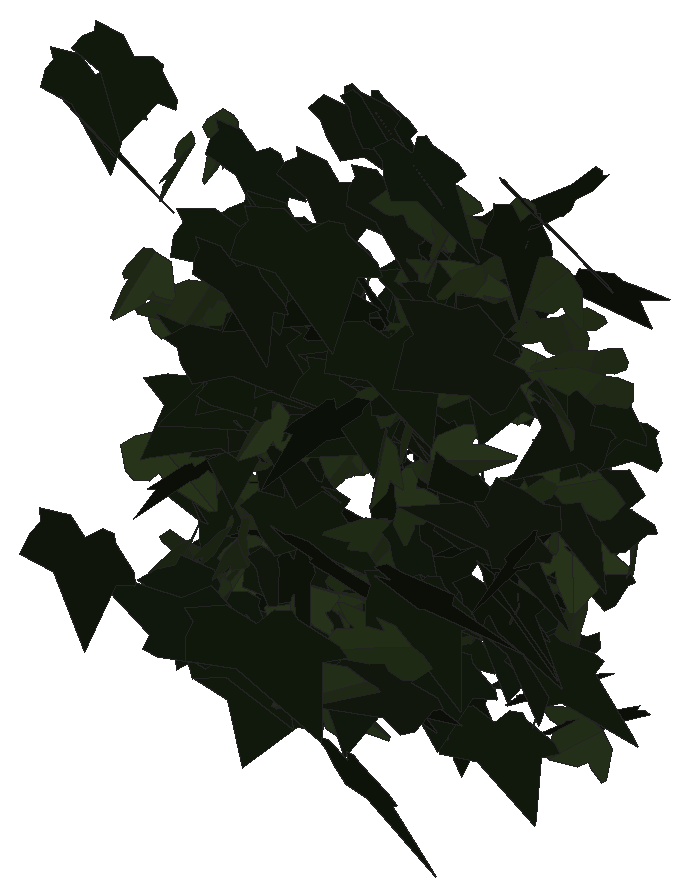
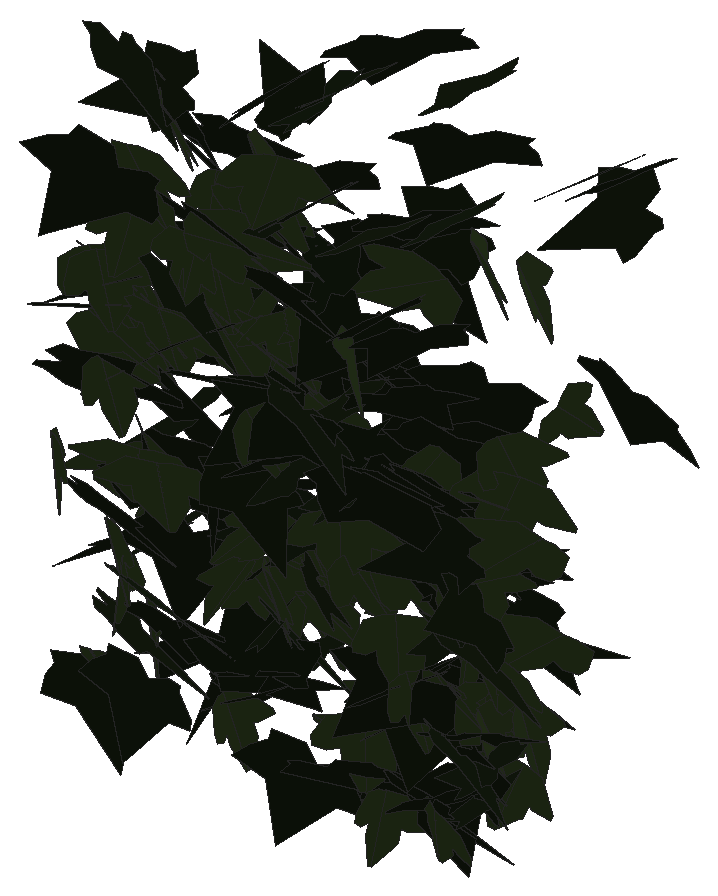
# SketchUp Ruby script. Lengths in millimetres.
U = 1.mm
M = Sketchup.active_model
def pt(a) = Geom::Point3d.new(a.map { |v| v * U })
def face(e, loops, mat)
  f = e.add_face(loops[0].map { |a| pt(a) })
  loops[1..].each { |l| e.add_face(l.map { |a| pt(a) }).erase! }
  f.material = f.back_material = mat if mat
  f
end
# faces: each face lists its corners as indices into pts; further lists are holes
def faces(e, pts, list, mat = nil) = list.each { |f| face(e, (f[0].is_a?(Array) ? f : [f]).map { |l| l.map { |i| pts[i] } }, mat) }
# xy, xz, yz: faces in a plane at the given z, y or x. An outline is a flat list of corners, or four numbers for a rectangle; further outlines are holes
def ring(l) = l.size == 4 ? [[l[0], l[1]], [l[2], l[1]], [l[2], l[3]], [l[0], l[3]]] : l.each_slice(2).to_a
def flat(e, list, mat, &to3) = list.each { |f| face(e, (f[0].is_a?(Array) ? f : [f]).map { |l| ring(l).map { |u, v| to3.(u, v) } }, mat) }
def xy(e, z, list, mat = nil) = flat(e, list, mat) { |x, y| [x, y, z] }
def xz(e, y, list, mat = nil) = flat(e, list, mat) { |x, z| [x, y, z] }
def yz(e, x, list, mat = nil) = flat(e, list, mat) { |y, z| [x, y, z] }
def lines(e, pts, list) = list.each { |a, b| e.add_line(pt(pts[a]), pt(pts[b])) }
# prism: a flat outline (further loops are holes) pulled along v
def prism(e, loops, v, mat = nil)
  f = face(e, loops, mat); d = Geom::Vector3d.new(v.map { |x| x * U })
  f.pushpull(f.normal.samedirection?(d) ? d.length : -d.length)
end
def box(e, o, s, mat = nil) = prism(e, [[o, [o[0] + s[0], o[1], o[2]], [o[0] + s[0], o[1] + s[1], o[2]], [o[0], o[1] + s[1], o[2]]]], [0, 0, s[2]], mat)
def at(x, y, z, deg = 0) = Geom::Transformation.translation(pt([x, y, z])) * Geom::Transformation.rotation(ORIGIN, Z_AXIS, deg.degrees)
def axes(o, x, y, z) = Geom::Transformation.new([*x, 0, *y, 0, *z, 0, *pt(o).to_a, 1])
def part(name) = M.definitions.add(name)
# library, detail: a bought-in or finely detailed component or shape, given as its bounding box
def library(name, o, s) = part(name).tap { |d| box(d.entities, o, s) }
def detail(e, o, s) = box(e.add_group.entities, o, s)
def put(e, d, t, mat = nil) = e.add_instance(d, t).tap { |i| i.material = mat if mat }
def group(e, t, mat = nil) = e.add_group.tap { |g| g.transformation = t; g.material = mat if mat }.entities
root = M.entities
M.materials.add("efeu1").color = [18, 25, 13]
M.materials.add("efeu2").color = [43, 57, 29]
c1 = part("ivyleaf_9")
p = [[39.1,54.8,31.7],[34.5,51.8,30.2],[-5.3,25.2,17.3],[-17.9,28.3,20.9],[-21.6,21.7,17],[-20.2,4.3,5.3],
  [-22.9,-0.3,2.5],[-17.1,-4,-0.6],[-2,-2.1,-1.2],[-0.7,-15.4,-10.1],[16.6,-22.3,-16.7],[21.1,-15.1,-12.5],
  [32.7,-10.7,-11],[46.1,-1.8,-6.6],[30.8,11.2,3.8]]
faces(c1.entities,p,[[0,1,2,3,4,5,6,7,8,9,10,11,12,13,14]],"efeu1")
c2 = part("ivyleaf_10")
p = [[0,12.8,-0.8],[-1.5,51.3,-10.9],[-4.9,51,-11.6],[-13.6,26.5,-7.3],[-13.2,15.9,-4.6],[-21.1,19.3,-7.2],
  [-29.5,16.3,-8.3],[-29.2,8.3,-6.2],[-19.7,-9.8,0.5],[-7.6,-13,4],[1,-12.2,5.8],[-0.4,51.1,-11.1],
  [-1.5,51.1,-10.9],[1,-12.4,5.9],[16.9,-12.4,3.5],[35.1,9.1,-5.1],[35,12.9,-6.1],[20.5,16.4,-4.9],
  [15.8,15,-3.8],[15.3,27.6,-7.1],[12.8,31.3,-7.8]]
faces(c2.entities,p,[[0,1,2,3,4,5,6,7,8,9,10],[11,12,0,13,14,15,16,17,18,19,20]],"efeu2")
put(root,c1,axes([5237.9,577.4,4146.6],[-0.22791,-1.24972,0.09422],[0.02085,-0.09569,-1.25528],[2.38512,-0.11858,0.01998]))
put(root,c2,axes([5260,640.4,3904.9],[0.32495,0.86733,-0.87553],[-0.70025,-0.8077,-0.87189],[-2.23853,0.37857,0.14565]))
put(root,c2,axes([5229.3,734.7,3803.5],[1.58084,0.45329,0.72541],[0.88096,0.61211,-0.91251],[-1.36903,0.91732,0.25045]))
put(root,c1,axes([5283.3,771.9,3561.8],[-0.28505,0.88899,0.74331],[-0.55358,0.69665,-0.8918],[-2.13482,-0.29935,0.13201]))
put(root,c2,axes([5256.9,721.9,3528.2],[-2.06429,0.48857,-0.04164],[0.07361,-0.01551,-1.1896],[-0.93031,-1.08533,-0.00174]))
put(root,c1,axes([5222.2,565.3,4111.4],[2.16937,-0.84957,-0.16786],[-0.25536,0.10087,-1.42163],[1.62825,1.14772,0.00069]))
put(root,c1,axes([5262.4,765.3,3729.2],[-0.69052,0.7987,-0.78771],[-0.61651,0.71802,0.87725],[2.04404,0.48638,-0.00151]))
put(root,c1,axes([5296.8,748.8,3676.6],[-0.56219,1.05041,0.51491],[-0.85878,0.38767,-1.04969],[-2.05412,-0.44956,0.29793]))
put(root,c1,axes([5254,619.8,4155.6],[-0.55085,-1.1448,0.445],[-0.10585,-0.44451,-1.1797],[2.33521,-0.29019,0.0515]))
put(root,c1,axes([5238.6,773.1,3564.9],[0.83099,-1.07671,0.08982],[0.09229,-0.07725,-1.16176],[2.05424,0.43902,0.01586]))
put(root,c2,axes([5275.1,676.9,3563.8],[0.02012,-1.23367,-0.11013],[0.02819,0.11025,-1.23362],[2.35709,0.00921,0.01569]))
put(root,c2,axes([5258.7,740.4,3658.2],[1.95897,-0.54814,0.29844],[0.5704,-0.07079,-1.16368],[1.04191,1.06935,0.07594]))
put(root,c2,axes([5245,678.7,3666.5],[1.70086,0.46056,0.67156],[1.03285,0.40653,-1.00099],[-1.15545,1.04134,0.09377]))
put(root,c1,axes([5297.6,735,3519.5],[-0.05382,-0.04278,1.25851],[-0.35098,1.24539,0.03819],[-2.37073,-0.18341,-0.03422]))
put(root,c2,axes([5274.2,701.9,3833.2],[-2.01706,-0.54132,-0.28818],[0.50917,0.10963,-1.18984],[1.05021,-1.09282,0.02338]))
put(root,c2,axes([5290.9,688.3,3864.9],[-0.85724,-1.10615,0.30759],[-0.12733,-0.30457,-1.19324],[2.18139,-0.45247,0.05123]))
put(root,c1,axes([5302.6,657.7,3674.5],[-0.53119,0.9267,-0.67379],[0.35509,-0.64747,-0.96779],[-2.1515,-0.33566,0.00662]))
put(root,c1,axes([5262,748.6,3515],[1.01788,-1.02385,-0.13399],[-0.1015,0.1233,-1.15508],[1.96258,0.53739,0.00975]))
put(root,c2,axes([5294.4,714,3568.3],[0.32806,-1.18206,0.10636],[-0.01479,-0.1086,-1.19434],[2.25875,0.17097,-0.02327]))
put(root,c2,axes([5294.2,651.9,4045.9],[0.53757,-1.20475,0.05693],[-0.00656,-0.05928,-1.23731],[2.29544,0.28197,-0.01687]))
put(root,c1,axes([5297,758,3574.9],[-1.55311,-0.84941,0.16483],[0.11329,-0.28115,-1.15413],[1.64285,-0.78362,0.23541]))
put(root,c2,axes([5304.1,727.2,3737],[-1.14837,-1.02735,0.23072],[0.10429,-0.29619,-1.17559],[2.00123,-0.57409,0.19365]))
put(root,c1,axes([5312.2,686,3734.8],[-1.35491,-0.79199,0.51244],[-0.71641,-0.35015,-1.06412],[1.64618,-0.80424,-0.04133]))
put(root,c1,axes([5308.1,709.1,3720],[-0.72384,-1.20414,-0.13162],[0.05169,0.12944,-1.26271],[2.30479,-0.38108,-0.01302]))
put(root,c1,axes([5313.1,775.2,3507],[-0.76161,-1.08531,0.1492],[-0.01712,-0.15558,-1.15586],[2.08492,-0.39774,0.04501]))
put(root,c2,axes([5306.3,775.9,3483.8],[1.58972,-0.71026,0.39583],[0.67689,-0.19116,-1.09353],[1.39162,0.90435,0.07972]))
put(root,c2,axes([5294.8,751.8,3594.9],[-0.20029,-0.10752,-1.16255],[1.26411,-0.96548,0.02917],[-1.82739,-0.65609,0.14759]))
put(root,c2,axes([5333.9,662.1,3545.3],[-0.46592,-1.18275,-0.22608],[0.02743,0.22781,-1.20741],[2.2916,-0.2432,-0.03152]))
put(root,c2,axes([5329.3,679.8,4070.3],[1.17842,-1.08302,0.07791],[0.05266,-0.07392,-1.24746],[2.06586,0.61967,-0.01264]))
put(root,c1,axes([5297.9,751.5,3775.4],[1.91409,-0.61192,0.16135],[0.28467,-0.06454,-1.17704],[1.17028,1.01654,0.0224]))
put(root,c1,axes([5362.8,700.6,3760.9],[-2.13188,-0.20027,0.3169],[-0.47549,-0.34563,-1.10155],[0.53192,-1.11163,0.2854]))
put(root,c1,axes([5351.3,736.2,3500],[1.07349,0.74499,-0.75413],[-0.92255,-0.57843,-0.93398],[-1.79421,0.74315,0.02904]))
put(root,c1,axes([5309.7,746.8,3684.9],[1.36334,-0.94,-0.05223],[-0.01949,0.05784,-1.18153],[1.79165,0.71591,0.02689]))
put(root,c1,axes([5359.2,713.3,3802.1],[-2.01308,-0.53843,0.06073],[-0.08795,-0.04308,-1.18676],[1.02748,-1.0586,0.01741]))
put(root,c2,axes([5350,762.8,3610.4],[-0.61426,-1.13811,0.01923],[0.01503,-0.02223,-1.18291],[2.16631,-0.32256,0.01366]))
put(root,c1,axes([5381.2,750.1,3484.8],[-1.9941,0.3785,0.34047],[-0.62301,0.09577,-1.11385],[-0.74206,-1.09752,0.02022]))
put(root,c2,axes([5367.8,651.2,3523],[-1.86562,0.27387,0.58187],[-1.05635,0.17549,-1.01765],[-0.61821,-1.12635,-0.01707]))
put(root,c2,axes([5350.5,704.1,3569.3],[0.84989,0.84491,-0.76393],[-0.67227,-0.67737,-0.95566],[-2.06099,0.56937,-0.0033]))
put(root,c1,axes([5368.1,703.7,3750.5],[-2.20645,-0.2236,-0.0257],[0.04676,0.00828,-1.1807],[0.4258,-1.15959,-0.00348]))
put(root,c1,axes([5357.6,633.8,3556.1],[-2.10836,-0.30583,-0.39696],[0.72036,0.12054,-1.14914],[0.62501,-1.17058,-0.01463]))
put(root,c1,axes([5354.9,738.5,3579.9],[1.2446,0.96259,-0.06883],[-0.31878,0.03132,-1.15323],[-1.80881,0.65682,0.15588]))
put(root,c1,axes([5389.9,731.6,3824.5],[-2.25643,0.12473,0.03765],[-0.08238,-0.05197,-1.19082],[-0.23389,-1.18506,0.05619]))
put(root,c1,axes([5408,547.4,3556.7],[-0.49827,0.40964,1.0866],[-2.04939,0.33134,-0.38436],[-0.82735,-1.06746,0.29768]))
put(root,c2,axes([5365.3,650.7,3611.4],[0.00245,-0.96061,-0.67602],[0.22173,0.67279,-0.9558],[2.22454,-0.066,0.09601]))
put(root,c2,axes([5389.3,720.3,3709.7],[-1.23799,-0.7406,0.69449],[-0.87674,-0.51972,-0.9857],[1.72194,-0.79707,-0.00257]))
put(root,c1,axes([5409.6,646.5,3801.2],[-0.02836,0.32803,1.17932],[-2.20002,0.38422,-0.12148],[-0.7664,-1.11507,0.30508]))
put(root,c2,axes([5376.1,756.2,3664.7],[-1.43593,-0.92194,-0.00246],[0.18958,-0.07835,-1.18455],[1.74437,-0.7504,0.12671]))
put(root,c2,axes([5374.1,613.7,3563.7],[0.76655,-1.1928,0.12568],[0.07356,-0.1196,-1.25897],[2.28152,0.40461,-0.00163]))
put(root,c2,axes([5372.8,778.4,3477.4],[-0.63948,-0.99066,-0.48377],[0.35537,0.4473,-1.04566],[2.0679,-0.38322,0.03009]))
put(root,c1,axes([5351,756,3616.3],[2.21156,0.28427,-0.00735],[-0.01443,0.00005,-1.19628],[-0.54101,1.16204,0.00185]))
put(root,c1,axes([5372.8,725.7,3704.2],[-1.82188,0.09461,-0.72432],[1.37764,-0.03746,-0.96155],[-0.18667,-1.19983,-0.0271]))
put(root,c1,axes([5365.5,761.6,3607.2],[0.38947,-1.08175,-0.44392],[0.04961,0.45477,-1.09618],[2.22484,0.17923,0.10215]))
put(root,c2,axes([5396,674.5,3763.6],[0.22483,0.57585,-1.08771],[-0.51037,-1.05441,-0.58734],[-2.28606,0.29204,0.02415]))
put(root,c2,axes([5383.9,686.5,3818.8],[-0.44911,-0.78626,-0.90793],[0.88728,0.79277,-0.80771],[2.10662,-0.50153,0.14663]))
put(root,c1,axes([5426.4,742.1,3814.4],[0.18199,0.71603,-0.96847],[-1.04944,-0.8377,-0.67379],[-2.03792,0.49532,0.26048]))
put(root,c1,axes([5379,722.6,3552.7],[-0.00877,-1.26429,-0.03826],[0.00435,0.03825,-1.2643],[2.40729,-0.00467,0.00215]))
put(root,c1,axes([5379.6,614.9,3878.1],[-0.15167,-0.47823,-1.25039],[0.56377,1.21525,-0.48368],[2.4847,-0.30493,0.03342]))
put(root,c1,axes([5388.8,654.9,4075.5],[-0.10535,-1.23831,0.35809],[0.085,-0.36005,-1.23817],[2.45184,-0.04072,0.05831]))
put(root,c1,axes([5396.5,360.9,3751.1],[-1.84525,-0.06355,-1.07431],[2.04789,-0.03196,-0.96921],[0.03582,-1.44677,0.0686]))
put(root,c1,axes([5392,709.1,3703.5],[-0.61097,-0.91042,0.83619],[0.49317,-0.89429,-0.8742],[2.30038,-0.05008,0.4095]))
put(root,c2,axes([5419.9,753.6,3534.7],[-1.89089,-0.60302,0.01928],[-0.0396,-0.00288,-1.16219],[1.14758,-0.99371,-0.00834]))
put(root,c1,axes([5443.1,729.2,3800.5],[-2.29494,-0.1099,0.15137],[-0.28902,-0.00146,-1.21077],[0.20789,-1.2153,-0.01223]))
put(root,c1,axes([5396,693.4,3581.1],[0.7215,-1.02551,-0.53719],[-0.12805,0.54478,-1.08749],[2.19959,0.3681,0.1129]))
put(root,c1,axes([5408.6,585.4,3544.7],[0.09476,-0.9833,-0.74105],[0.07131,0.74252,-0.98273],[2.34226,0.01718,0.0599]))
put(root,c2,axes([5440.4,738.2,3703.4],[-0.8309,-1.01558,0.47968],[-0.1626,-0.48313,-1.10063],[2.13141,-0.43276,0.10303]))
put(root,c1,axes([5413.7,681.5,3954],[-0.23004,-1.09468,-0.56798],[0.13159,0.56379,-1.10132],[2.34345,-0.13911,0.00609]))
put(root,c1,axes([5441.9,686.1,3876],[-1.59733,-0.89633,0.20818],[-0.30492,-0.13512,-1.22769],[1.72455,-0.8541,-0.02425]))
put(root,c1,axes([5442.9,777.7,3496.4],[-1.63597,-0.77741,-0.01579],[0.03221,0.00483,-1.15896],[1.47952,-0.85972,0.00777]))
put(root,c2,axes([5419.6,687.2,3541.6],[1.21661,0.72765,0.69517],[0.44629,0.69319,-0.9412],[-1.86255,0.64139,0.22856]))
put(root,c2,axes([5438.9,618.6,3512.1],[0.49921,-1.00435,0.55414],[0.47723,-0.50449,-1.03306],[2.13032,0.34837,0.10157]))
put(root,c1,axes([5452.7,601.3,3495.1],[-1.26317,-1.0191,0.02927],[-0.03828,-0.02184,-1.21617],[1.93998,-0.66399,-0.00493]))
put(root,c2,axes([5457.8,744.8,3748.8],[-1.78084,-0.76233,0.03479],[0.2411,-0.20945,-1.18237],[1.43223,-0.91263,0.24229]))
put(root,c1,axes([5423.6,663.8,3674.7],[0.69608,-0.87243,-0.82538],[0.40114,0.89604,-0.85372],[2.25026,0.11014,0.40751]))
put(root,c1,axes([5440,702.4,3974.9],[0.27596,-1.21425,-0.24147],[-0.05558,0.2397,-1.22288],[2.35556,0.14791,-0.00057]))
put(root,c1,axes([5441,740.4,3792.7],[0.84382,-1.13121,0.01637],[0.00249,-0.01707,-1.21499],[2.15315,0.44334,-0.00501]))
put(root,c1,axes([5435.8,577.7,4019.5],[2.39168,-0.52278,-0.12136],[-0.21303,0.0469,-1.36107],[0.99896,1.26164,0.00031]))
put(root,c2,axes([5493.6,684.7,3909.1],[-0.09238,0.68487,0.99138],[-1.41521,0.76369,-0.56398],[-1.80447,-0.63401,0.39157]))
put(root,c1,axes([5471.6,615.7,4035.2],[-1.36968,-1.05973,-0.05846],[0.0738,0.04433,-1.28098],[2.0186,-0.72068,0.00717]))
put(root,c1,axes([5463.9,695.3,4047.6],[-0.54818,-1.14377,0.45283],[0.11547,-0.47772,-1.16804],[2.33836,-0.24454,0.16383]))
put(root,c2,axes([5450.4,620.7,3974.5],[-1.66533,0.28806,-0.84956],[1.54659,-0.24813,-0.92111],[-0.72312,-1.19408,-0.01354]))
put(root,c1,axes([5496.6,716.9,3778.1],[-1.55553,-0.66662,0.5649],[-0.61723,-0.48682,-1.04371],[1.54418,-0.8661,0.15187]))
put(root,c1,axes([5479.4,759.5,3476.6],[1.28471,0.94644,0.089],[0.08238,0.07844,-1.16246],[-1.80734,0.67634,0.01028]))
put(root,c1,axes([5511.9,591.3,3988.4],[0.75224,0.52275,-1.20226],[-1.26302,-1.00316,-0.65436],[-2.15178,0.77157,-0.03622]))
put(root,c1,axes([5517.6,724.2,3848.1],[-0.18634,1.03475,0.63578],[-0.46193,0.6083,-1.02741],[-2.26474,-0.20921,0.15725]))
put(root,c1,axes([5468.9,617.5,3637.4],[-0.4806,-0.17771,-1.14255],[2.07869,-0.42056,-0.17598],[-0.7224,-1.09193,0.25373]))
put(root,c1,axes([5480.3,514.2,4079.6],[-0.90272,-0.99512,-0.72011],[0.60351,0.64657,-1.10236],[2.25854,-0.57051,0.00674]))
put(root,c2,axes([5455,674.4,3458.3],[-0.03992,-0.11471,1.23716],[2.31706,-0.24892,-0.00244],[0.47208,1.21204,0.11659]))
put(root,c2,axes([5492.1,605.5,3596.8],[-0.11916,1.13127,0.37431],[-0.01184,0.37451,-1.13292],[-2.2678,-0.0614,-0.01375]))
put(root,c2,axes([5519,714.6,3634.9],[-1.13193,-0.77398,0.67122],[-0.34215,-0.68524,-0.94944],[1.91955,-0.57854,0.22658]))
put(root,c1,axes([5509.8,730.9,3676.5],[-1.33174,0.44726,-0.83712],[1.2696,-0.50805,-0.82905],[-1.28491,-0.96555,0.04846]))
put(root,c2,axes([5523.3,694.2,3663.9],[-0.97706,-1.07875,0.23056],[-0.13089,-0.22251,-1.19423],[2.09537,-0.51692,0.03291]))
put(root,c1,axes([5491.2,675.7,3847.5],[1.25146,-1.008,-0.38591],[-0.10607,0.41957,-1.1909],[2.05148,0.63661,0.17384]))
put(root,c1,axes([5551.4,726.3,3611.6],[-1.60967,0.82767,-0.03501],[0.03983,-0.02868,-1.18336],[-1.57613,-0.84601,0.00586]))
put(root,c1,axes([5537.2,773.7,3563.1],[-1.72545,-0.72803,0.12405],[-0.08938,-0.13918,-1.16008],[1.40272,-0.90441,0.07867]))
put(root,c1,axes([5517.8,643,3922.4],[1.54915,0.88754,0.23094],[0.27093,0.18276,-1.20414],[-1.72426,0.82612,0.01828]))
put(root,c1,axes([5543,588.4,3855.2],[-0.59743,0.82169,-1.14209],[0.80672,-1.06057,-0.87954],[-2.55331,-0.52735,-0.01066]))
put(root,c2,axes([5536.5,751.7,3659.3],[1.06882,-1.05252,-0.11899],[0.01195,0.13799,-1.1909],[2.01587,0.55723,0.07015]))
put(root,c1,axes([5508.1,737.4,3725.4],[1.53365,-0.90449,0.13717],[0.30048,-0.04255,-1.20811],[1.71498,0.81631,0.08901]))
put(root,c1,axes([5533.2,644.9,3860.2],[-0.86568,-1.05863,-0.34168],[0.33066,0.297,-1.15149],[2.09114,-0.48521,0.04063]))
put(root,c2,axes([5569.5,740.8,3652.1],[-1.49094,-0.75221,0.50739],[-0.67515,-0.36306,-1.08596],[1.5894,-0.85984,0.01466]))
put(root,c1,axes([5516.4,742.1,3782.7],[0.82108,-1.11758,0.19461],[0.38181,-0.12976,-1.18991],[2.12495,0.45515,0.13861]))
put(root,c1,axes([5528.4,721.7,3841.7],[2.22595,0.32562,0.09535],[0.13299,0.10374,-1.21136],[-0.63191,1.16887,0.08095]))
put(root,c1,axes([5523.2,640.4,4181.8],[1.01346,-1.0837,-0.55234],[0.00125,0.60321,-1.18287],[2.31494,0.47411,0.24245]))
put(root,c1,axes([5535.4,695.4,4063.3],[0.03492,-1.25886,0.08215],[-0.07644,-0.0827,-1.25832],[2.39974,0.01569,-0.04128]))
put(root,c1,axes([5534.7,743.1,3622.4],[1.31326,-0.8234,-0.47872],[-0.61211,0.35499,-1.07417],[1.70623,0.76111,-0.0169]))
put(root,c1,axes([5526.8,773.6,3575.1],[2.36028,-0.40697,-0.16293],[0.29799,-0.04543,1.30522],[-0.77928,-1.25,0.00561]))
put(root,c1,axes([5529.6,678.3,3552.1],[0.61074,-1.15031,0.18653],[0.09004,-0.18045,-1.19422],[2.21603,0.32436,-0.00289]))
put(root,c1,axes([5532.7,443.5,4082.3],[0.08081,-1.24525,0.32852],[0.18294,-0.32472,-1.24326],[2.44421,0.06548,0.08219]))
put(root,c1,axes([5572.3,748.8,3766.8],[0.01859,1.16074,-0.31388],[-0.01554,-0.31382,-1.16077],[-2.28842,0.01156,0.00533]))
put(root,c1,axes([5532.2,666.9,3956.8],[0.10545,-0.69373,1.06934],[0.3346,-1.05596,-0.69416],[2.40274,0.1775,0.04973]))
put(root,c2,axes([5566.3,739.2,3822.3],[-0.44659,-1.13394,0.36765],[0.00431,-0.37513,-1.15556],[2.2687,-0.2225,0.07457]))
put(root,c2,axes([5543.8,745.3,3722.7],[-0.89075,-0.69567,-0.84847],[1.16576,0.59965,-0.82954],[1.7325,-0.76116,0.12194]))
put(root,c1,axes([5533.6,667.8,4173.2],[1.00733,-1.17601,-0.19376],[-0.11767,0.18463,-1.28949],[2.26531,0.53254,0.01918]))
put(root,c1,axes([5542.7,737,3791.1],[-0.02128,-1.15401,-0.32636],[0.05407,0.32602,-1.15381],[2.28181,-0.01849,0.0243]))
put(root,c1,axes([5610.5,632.4,3898],[-1.57971,0.81696,0.59511],[-0.91206,0.35991,-1.16247],[-1.69367,-0.95581,0.07094]))
put(root,c1,axes([5556.4,758.2,3528.9],[-0.66879,-1.1043,0.19735],[0.07828,-0.21935,-1.15416],[2.13356,-0.33811,0.10421]))
put(root,c2,axes([5573.1,770.8,3513.6],[-0.26119,-1.1541,0.02566],[0.02357,-0.02731,-1.16213],[2.1969,-0.13692,0.01552]))
put(root,c1,axes([5554.6,706.1,3666.9],[0.74374,-0.9301,-0.68902],[-0.52012,0.63253,-1.00885],[2.14071,0.47683,-0.00573]))
put(root,c1,axes([5604,713.1,3980.1],[-2.29641,0.19295,-0.0226],[0.04154,-0.0066,-1.22193],[-0.3674,-1.2068,0.00307]))
put(root,c2,axes([5576.4,687.1,3916.2],[0.61752,1.12014,-0.30063],[-0.44513,-0.24256,-1.15621],[-2.16194,0.36989,0.15219]))
put(root,c2,axes([5572.9,762.8,3666.2],[0.09929,1.04428,0.55607],[-0.09521,0.55806,-1.04332],[-2.24967,0.02247,0.0687]))
put(root,c1,axes([5566.5,587.8,3561.3],[-0.50327,-1.25582,0.57352],[-0.0107,-0.58296,-1.27908],[2.6275,-0.24291,0.10465]))
put(root,c2,axes([5626.5,736.6,4012.1],[-0.10736,-0.0053,-1.21676],[-2.30349,0.12553,0.05557],[0.23819,1.21159,-0.01108]))
put(root,c1,axes([5596.3,721.1,3905.3],[-2.14262,0.09096,-0.51064],[0.89211,-0.344,-1.09471],[-0.42261,-1.18736,0.27804]))
put(root,c2,axes([5580.4,679.6,3841.6],[0.59218,-1.07411,0.59459],[0.55023,-0.53204,-1.1124],[2.27086,0.40901,0.11448]))
put(root,c2,axes([5594.3,648.6,3879.6],[-0.59212,-1.18985,0.25359],[0.0115,-0.26326,-1.2278],[2.31535,-0.30298,0.07095]))
put(root,c2,axes([5586.3,688.5,4079.5],[-1.68105,-0.85832,-0.26691],[0.62259,0.04158,-1.2163],[1.5934,-0.92179,0.19366]))
put(root,c1,axes([5545.8,557.3,3695.3],[0.69986,-0.69134,0.97636],[1.54889,-0.60413,-0.73428],[1.66887,0.85061,0.27204]))
put(root,c2,axes([5596.2,610.4,3555.5],[1.73628,-0.80986,-0.22247],[-0.25214,0.18559,-1.21888],[1.57842,0.92051,0.05001]))
put(root,c1,axes([5613.3,663.9,4001.9],[-1.94195,0.27097,-0.61037],[1.06532,-0.26083,-1.05155],[-0.69316,-1.16002,0.09387]))
put(root,c1,axes([5579.2,664.3,4136.4],[0.05047,-0.58453,1.12018],[0.50563,-1.0928,-0.57653],[2.35097,0.24758,0.09995]))
put(root,c1,axes([5583.3,415,3690.5],[-1.09596,-0.84006,-1.0577],[1.0808,0.89268,-1.01817],[2.33244,-0.80837,-0.02519]))
put(root,c2,axes([5601.8,630.7,3748.8],[0.2937,-0.4838,-1.0836],[0.65532,1.06397,-0.42599],[2.16135,-0.25685,0.27641]))
put(root,c1,axes([5597.9,477,4131.2],[-0.74936,-1.36873,-0.41622],[0.23072,0.39822,-1.42423],[2.71296,-0.41193,0.00615]))
put(root,c1,axes([5621.7,740.8,3858.4],[-1.84968,-0.72677,0.06942],[0.30589,-0.32573,-1.16001],[1.3554,-0.91829,0.35653]))
put(root,c2,axes([5639.6,706.9,3892.6],[-1.71194,-0.62224,0.52279],[-0.60498,-0.44833,-1.08054],[1.42352,-0.93884,0.1695]))
put(root,c1,axes([5630.9,677.6,3969.9],[-1.60025,-0.7293,0.5622],[-0.24376,-0.66129,-1.04939],[1.73551,-0.76534,0.37099]))
put(root,c1,axes([5617,703.4,3695.5],[-1.63112,0.08996,-0.83444],[1.57096,-0.1254,-0.8613],[-0.28895,-1.18957,0.02769]))
put(root,c2,axes([5654.2,472.9,3623.2],[-1.0201,-0.61099,0.90996],[-1.2009,-0.65624,-0.8123],[1.70567,-0.82745,-0.02769]))
put(root,c1,axes([5637.5,724,3678.4],[-0.02862,-0.29707,1.22609],[0.33437,1.21374,0.29623],[-2.37762,0.17427,0.0269]))
put(root,c2,axes([5622.1,578.7,3841.7],[-0.05744,0.68288,-1.05586],[-0.06864,-1.0562,-0.68206],[-2.39218,0.01391,0.04492]))
put(root,c1,axes([5606.2,644.5,4152.4],[0.65619,-1.19798,-0.46052],[-0.20203,0.4486,-1.24644],[2.43429,0.36016,0.02069]))
put(root,c2,axes([5635,652.1,4067.1],[0.71939,-1.17516,-0.2445],[-0.06562,0.2456,-1.23376],[2.28352,0.37728,0.04157]))
put(root,c2,axes([5669.8,585,3977.4],[-1.16962,0.30427,1.06178],[-1.94107,0.3101,-0.67918],[-0.80694,-1.18697,0.09474]))
put(root,c1,axes([5659.3,728.9,4025.2],[-2.27947,0.20963,-0.20521],[0.37401,-0.06709,-1.2155],[-0.41452,-1.2133,0.03176]))
put(root,c2,axes([5646.7,700.7,3954.9],[-1.19833,-1.06262,0.0762],[-0.06167,-0.06937,-1.23513],[2.02663,-0.63043,0.00747]))
put(root,c1,axes([5634.6,640.9,3572.6],[-1.65433,-0.51725,-0.66424],[1.11773,0.31152,-1.01113],[1.14801,-1.04868,0.02727]))
put(root,c2,axes([5630.7,665.2,4014.4],[-2.03574,-0.32937,-0.48835],[1.03621,-0.16648,-1.08025],[0.42784,-1.164,0.29269]))
put(root,c1,axes([5606.8,584.3,3568],[0.295,-0.57797,1.27547],[1.31156,-1.08563,-0.57569],[2.32001,0.68722,0.16327]))
put(root,c1,axes([5622.1,699.2,3998.6],[-0.03702,-0.96662,0.79334],[0.69716,-0.76303,-0.92072],[2.27554,0.21805,0.29499]))
put(root,c1,axes([5651.9,666.7,3504.5],[0.71278,-0.5041,-1.20181],[-1.41953,0.9425,-0.62777],[2.03397,0.83444,-0.01697]))
put(root,c2,axes([5660.9,727.5,3980],[-1.80082,0.75703,0.10768],[-0.25934,0.00164,-1.2089],[-1.43199,-0.95231,0.08352]))
put(root,c1,axes([5661.2,724.8,3658.1],[1.79824,0.27481,-0.69298],[-1.31091,-0.10609,-0.98122],[-0.54267,1.16692,0.07399]))
put(root,c1,axes([5654,758.6,3577.9],[-1.74966,-0.4524,-0.5769],[1.11007,0.10923,-1.01514],[0.84532,-1.07983,0.139]))
put(root,c1,axes([5656.3,724.5,3883.8],[-0.72661,-1.06436,0.43406],[-0.13948,-0.4339,-1.12844],[2.18321,-0.38196,0.07237]))
put(root,c1,axes([5689.7,722.4,3944.2],[-1.05703,1.09572,-0.11493],[0.10917,-0.09978,-1.22843],[-2.09398,-0.55832,-0.00603]))
put(root,c1,axes([5702.6,770.7,3613.9],[-1.70823,0.71823,0.24274],[-0.57649,0.00511,-1.13517],[-1.32272,-0.92979,0.18127]))
put(root,c1,axes([5663.9,650.2,3978],[-0.89608,-0.78978,0.87312],[-0.11232,-0.92334,-0.86702],[2.23787,-0.36258,0.3061]))
put(root,c1,axes([5652.5,544.2,3995.2],[-0.5806,-1.13496,-0.64938],[0.31606,0.62779,-1.17524],[2.46848,-0.34733,-0.00226]))
put(root,c1,axes([5686,627.8,3944.1],[-1.98022,-0.55378,0.58314],[0.96947,0.28403,1.17862],[-1.18434,1.15843,-0.01022]))
put(root,c1,axes([5711,496.1,3635.3],[-2.40725,0.12897,0.36633],[-0.69893,0.00895,-1.27111],[-0.24053,-1.3168,0.02724]))
put(root,c2,axes([5669.9,673.7,4026.8],[-0.66278,-1.12211,-0.3218],[0.43959,0.26294,-1.16682],[2.17777,-0.39458,0.13759]))
put(root,c2,axes([5714.5,475.4,3689],[-1.33219,-0.11219,1.00129],[-1.81921,-0.31155,-0.70313],[0.6063,-1.18131,0.09035]))
put(root,c2,axes([5678.7,751.7,3733],[2.00244,0.54316,-0.08048],[-0.33065,0.1643,-1.16246],[-0.99133,1.04235,0.22517]))
put(root,c1,axes([5686,764.1,3502.1],[0.76478,1.06673,0.28976],[0.19462,0.27112,-1.13991],[-2.09475,0.41465,-0.00012]))
put(root,c2,axes([5687.8,731.9,3895.7],[2.31861,-0.17816,-0.0046],[-0.00927,-0.00155,-1.23123],[0.33906,1.21828,-0.00223]))
put(root,c1,axes([5688,657.9,3724],[-1.60344,0.83191,0.63268],[0.81058,-0.46884,1.18362],[1.8165,0.94354,0.0303]))
put(root,c1,axes([5733.2,704.5,3715.3],[-0.26777,0.49418,-1.09361],[-1.12375,-0.98711,-0.37009],[-1.98842,0.49131,0.35643]))
put(root,c1,axes([5739.2,750.5,3558],[-1.66181,0.77355,-0.16763],[0.01077,-0.24349,-1.15307],[-1.50635,-0.85512,0.17669]))
put(root,c1,axes([5694.4,666.8,3502.8],[-0.36957,-1.12608,-0.4805],[0.23291,0.46621,-1.14206],[2.31844,-0.22634,0.03814]))
put(root,c1,axes([5709.5,605.4,3839.2],[-0.73031,-0.44349,1.32469],[-0.50187,-1.32607,-0.52033],[2.6109,-0.37895,0.27052]))
put(root,c1,axes([5746.4,605.6,4007.6],[-1.99224,0.63974,0.05111],[-0.08325,0.02645,-1.2268],[-1.2186,-1.0477,0.00024]))
put(root,c1,axes([5676.7,451.6,3545.2],[1.2417,-1.21456,0.37859],[0.37855,-0.32286,-1.37853],[2.39147,0.68173,0.02164]))
put(root,c2,axes([5722.9,708,3544],[0.59705,-0.91209,-0.72587],[-0.16345,0.73157,-0.95636],[2.21248,0.30018,0.12523]))
put(root,c2,axes([5711.7,691.9,4098.6],[1.25282,-0.99824,0.31042],[0.3094,-0.26462,-1.19571],[1.96539,0.67798,-0.00964]))
put(root,c2,axes([5704.4,753.9,3745],[2.05114,0.49298,0.08286],[0.15457,0.02163,-1.18505],[-0.93875,1.0807,-0.01408]))
put(root,c2,axes([5700.5,574.6,3863.1],[-0.37547,-0.22405,-1.23119],[1.31299,1.02041,-0.29624],[1.98707,-0.71659,-0.0369]))
put(root,c1,axes([5763.4,564.9,4010.7],[-2.72035,-0.00754,0.34111],[-0.64917,-0.00369,-1.42937],[0.01559,-1.46949,0.00184]))
put(root,c1,axes([5702.6,525.6,3724.1],[0.1102,-1.41968,-0.332],[-0.10684,0.32985,-1.42025],[2.77278,0.06913,-0.04153]))
put(root,c2,axes([5720.5,754.9,3608.7],[0.3178,-1.10158,-0.41446],[0.40735,0.44005,-1.08337],[2.20266,0.07756,0.26015]))
put(root,c2,axes([5720.1,712.6,3736.6],[1.5379,-0.87014,0.18251],[0.24192,-0.13102,-1.18747],[1.6747,0.81799,0.00394]))
put(root,c1,axes([5745.2,764.2,3487.1],[0.37638,1.15058,-0.17519],[-0.08544,-0.17003,-1.16735],[-2.21336,0.20222,0.01527]))
put(root,c2,axes([5741.7,744.7,3638.4],[0.9806,-0.91984,-0.56841],[-0.24889,0.57201,-1.04421],[2.04281,0.51124,0.14563]))
put(root,c2,axes([5747.8,698,4038.1],[1.87122,-0.5553,-0.55425],[-0.66992,0.48194,-1.10728],[1.33448,1.02059,0.22131]))
put(root,c2,axes([5735.8,658.7,3669.4],[-0.15914,-0.32402,-1.17252],[0.44079,1.14955,-0.33418],[2.27283,-0.24563,-0.01729]))
put(root,c1,axes([5724.1,670,4103],[-1.28439,-0.00221,-1.0844],[1.99946,-0.31785,-0.65316],[-0.51144,-1.23707,0.16976]))
put(root,c1,axes([5704,652.4,3671],[-0.44894,-0.21444,-1.17844],[2.24366,0.17097,-0.26709],[0.40338,-1.18959,0.17404]))
put(root,c1,axes([5713.3,654.3,3747],[1.03187,-1.14383,-0.20299],[-0.14231,0.18918,-1.26575],[2.20636,0.54715,0.0133]))
put(root,c1,axes([5771.3,753.8,3683.6],[-2.11212,0.39612,0.0108],[-0.01443,0.0109,-1.17833],[-0.75405,-1.10977,-0.00772]))
put(root,c1,axes([5713.3,665.3,3663.6],[0.56977,-1.00836,0.62481],[0.35219,-0.59681,-1.05184],[2.23002,0.35189,0.00648]))
put(root,c2,axes([5758.1,738.4,3483.6],[1.58551,-0.60202,-0.56378],[-0.81717,0.36764,-1.02703],[1.34028,0.93633,0.04076]))
put(root,c1,axes([5728.7,676.2,3616.9],[-0.0484,-1.18006,0.43503],[-0.04397,-0.4346,-1.18026],[2.39324,-0.03185,-0.01288]))
put(root,c1,axes([5702,495.4,3750.2],[2.04877,-0.25344,0.52385],[0.96496,-0.1322,-1.10586],[0.5436,1.18986,-0.01128]))
put(root,c1,axes([5712.7,682.2,4128.2],[1.80549,-0.8233,0.11988],[0.16263,-0.08443,-1.25607],[1.57505,0.95247,-0.00773]))
put(root,c2,axes([5749.5,706,3980.7],[-1.23561,-0.95307,-0.41336],[0.44435,0.34111,-1.15318],[1.92656,-0.68993,0.00086]))
put(root,c2,axes([5774.4,673.3,3888.5],[0.48844,-0.19691,-1.22474],[-1.02622,1.10863,-0.29123],[2.12615,0.58033,0.14079]))
put(root,c2,axes([5764.8,736.1,3930.7],[-1.13908,-1.06333,0.0383],[0.02113,-0.05018,-1.21972],[2.02493,-0.59763,0.03427]))
put(root,c1,axes([5783.9,682.3,4149.3],[-0.68338,1.18933,0.13807],[-0.11232,0.12639,-1.24219],[-2.27597,-0.36334,0.01985]))
put(root,c1,axes([5802.5,589.7,3800.8],[-1.00534,-0.12852,1.0872],[-2.00843,-0.26148,-0.54365],[0.55449,-1.18012,0.00205]))
put(root,c2,axes([5771.1,719.3,3802.1],[-0.60667,-1.15959,0.0107],[-0.00929,-0.00976,-1.2026],[2.207,-0.31879,-0.00212]))
put(root,c2,axes([5760.5,713,3712.1],[1.13982,1.02179,-0.16946],[-0.15279,-0.14937,-1.18436],[-1.96531,0.60422,-0.00621]))
put(root,c2,axes([5805,681.6,3824.4],[-1.52894,0.07999,0.91342],[-1.69531,-0.35606,-0.75224],[0.41382,-1.16316,0.29309]))
put(root,c2,axes([5785.9,714.9,3918.3],[-1.4916,-0.8716,0.41452],[-0.43211,-0.35249,-1.17045],[1.78532,-0.81352,0.06303]))
put(root,c2,axes([5770.8,617.6,3820.5],[-0.71505,-1.02996,-0.52044],[0.42189,0.47272,-1.09555],[2.15536,-0.43422,0.04179]))
put(root,c1,axes([5763.6,718.7,4033.8],[2.09477,0.5492,0.00749],[0.00969,0.00657,-1.23006],[-1.04529,1.10066,0.0036]))
put(root,c1,axes([5805.5,677.5,3891.5],[-2.11278,0.34119,-0.34354],[0.57967,-0.1759,-1.15892],[-0.71633,-1.14867,0.07542]))
put(root,c1,axes([5827.2,710.7,3788.3],[-1.89382,-0.14357,0.67013],[-1.2716,-0.05979,-1.00492],[0.29037,-1.19819,-0.03015]))
put(root,c1,axes([5767.9,685.2,3793.6],[0.32111,-1.18535,-0.2059],[-0.08043,0.20195,-1.19723],[2.28833,0.17343,-0.01318]))
put(root,c1,axes([5760.7,670.8,3604],[0.71853,-0.93176,-0.6916],[0.1802,0.74959,-0.95821],[2.20107,0.2428,0.30422]))
put(root,c1,axes([5781.5,725.6,3896.4],[-0.83768,-1.11623,0.28511],[0.01172,-0.30748,-1.19432],[2.19259,-0.42482,0.11531]))
put(root,c1,axes([5801.6,731.1,3873.5],[-1.66582,-0.80633,0.29196],[0.08024,-0.45713,-1.13612],[1.63014,-0.80148,0.35427]))
put(root,c2,axes([5800.8,761.4,3723.5],[0.81813,-1.04565,-0.35456],[0.14403,0.40749,-1.11001],[2.09644,0.38007,0.21462]))
put(root,c1,axes([5806.2,585.4,3793.5],[-0.77555,0.4158,-1.06374],[1.04189,-0.92012,-0.56937],[-1.90771,-0.67155,0.12149]))
